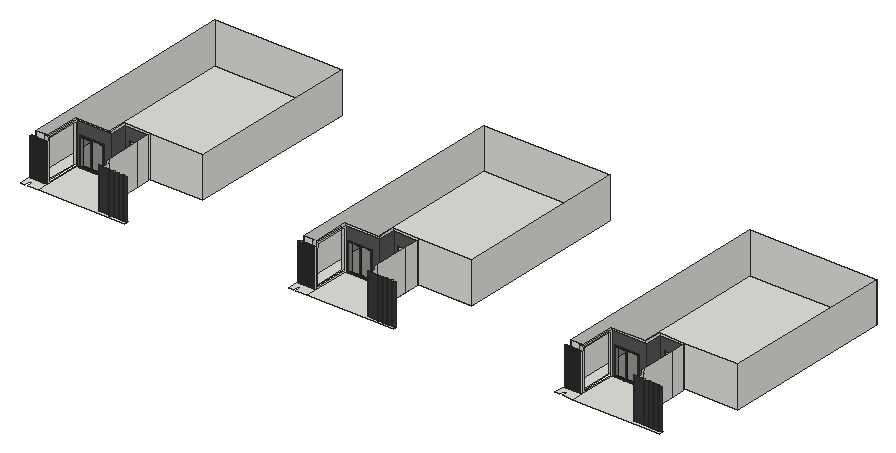
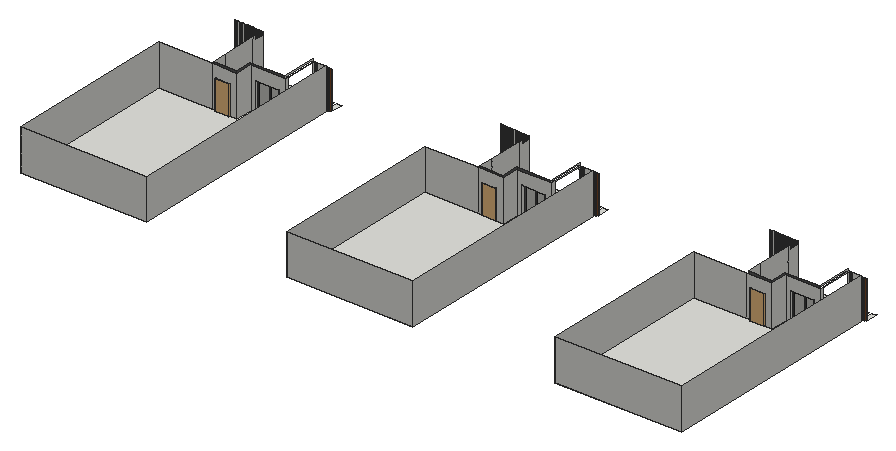
# SketchUp Ruby script. Lengths in inches.
U = 1.inch
M = Sketchup.active_model
def pt(a) = Geom::Point3d.new(a.map { |v| v * U })
def face(e, loops, mat)
  f = e.add_face(loops[0].map { |a| pt(a) })
  loops[1..].each { |l| e.add_face(l.map { |a| pt(a) }).erase! }
  f.material = f.back_material = mat if mat
  f
end
# faces: each face lists its corners as indices into pts; further lists are holes
def faces(e, pts, list, mat = nil) = list.each { |f| face(e, (f[0].is_a?(Array) ? f : [f]).map { |l| l.map { |i| pts[i] } }, mat) }
# xy, xz, yz: faces in a plane at the given z, y or x. An outline is a flat list of corners, or four numbers for a rectangle; further outlines are holes
def ring(l) = l.size == 4 ? [[l[0], l[1]], [l[2], l[1]], [l[2], l[3]], [l[0], l[3]]] : l.each_slice(2).to_a
def flat(e, list, mat, &to3) = list.each { |f| face(e, (f[0].is_a?(Array) ? f : [f]).map { |l| ring(l).map { |u, v| to3.(u, v) } }, mat) }
def xy(e, z, list, mat = nil) = flat(e, list, mat) { |x, y| [x, y, z] }
def xz(e, y, list, mat = nil) = flat(e, list, mat) { |x, z| [x, y, z] }
def yz(e, x, list, mat = nil) = flat(e, list, mat) { |y, z| [x, y, z] }
def lines(e, pts, list) = list.each { |a, b| e.add_line(pt(pts[a]), pt(pts[b])) }
# prism: a flat outline (further loops are holes) pulled along v
def prism(e, loops, v, mat = nil)
  f = face(e, loops, mat); d = Geom::Vector3d.new(v.map { |x| x * U })
  f.pushpull(f.normal.samedirection?(d) ? d.length : -d.length)
end
def box(e, o, s, mat = nil) = prism(e, [[o, [o[0] + s[0], o[1], o[2]], [o[0] + s[0], o[1] + s[1], o[2]], [o[0], o[1] + s[1], o[2]]]], [0, 0, s[2]], mat)
def at(x, y, z, deg = 0) = Geom::Transformation.translation(pt([x, y, z])) * Geom::Transformation.rotation(ORIGIN, Z_AXIS, deg.degrees)
def axes(o, x, y, z) = Geom::Transformation.new([*x, 0, *y, 0, *z, 0, *pt(o).to_a, 1])
def part(name) = M.definitions.add(name)
# library, detail: a bought-in or finely detailed component or shape, given as its bounding box
def library(name, o, s) = part(name).tap { |d| box(d.entities, o, s) }
def detail(e, o, s) = box(e.add_group.entities, o, s)
def put(e, d, t, mat = nil) = e.add_instance(d, t).tap { |i| i.material = mat if mat }
def group(e, t, mat = nil) = e.add_group.tap { |g| g.transformation = t; g.material = mat if mat }.entities
root = M.entities
M.materials.add("Glass_Tinted_Gray").color = [0, 0, 0]
M.materials["Glass_Tinted_Gray"].alpha = 0.125
M.materials.add("[0135_DarkGray]").color = [81, 81, 81]
M.materials.add("[Color M06]").color = [86, 86, 86]
M.materials.add("[Color M07]").color = [58, 58, 58]
M.materials.add("[Mirror 02]").color = [229, 229, 229]
M.materials.add("[Terrazzo Light Blue]").color = [196, 214, 227]
M.materials.add("[Wood Veneer 01]").color = [120, 70, 37]
c1 = part("PENTEK_RP Fineline 50S_Sliding_DoorCase_E1")
box(c1.entities,[0,0,0],[1.51,3.66,99.27],"[0135_DarkGray]")
c2 = part("PENTEK_RP Fineline 50S_SlidingDooe_Case_E2")
box(c2.entities,[0,0,0],[96.25,3.66,1.51],"[0135_DarkGray]")
c3 = part("pentek_RP Fineline 50S_SlidingDoor_Case")
put(c3.entities,c1,at(97.76,0,0))
put(c3.entities,c2,at(1.51,0,0))
put(c3.entities,c1,at(0,0,0))
put(c3.entities,c2,at(1.51,0,97.76))
c4 = part("PENTEK_RP Fineline 50S_SlidingDoor_GlazingBead_2")
box(c4.entities,[0,0,0],[0.56,0.59,94.39],"[0135_DarkGray]")
c5 = part("PENTEK_RP Fineline 50S_SlidingDoor_Glass")
box(c5.entities,[0,0,0],[46.58,0.16,94.39],"Glass_Tinted_Gray")
c6 = part("PENTEK_RP Fineline 50S_SlidingDoor_GlazingBead")
box(c6.entities,[0,0,0],[45.47,0.59,0.56],"[0135_DarkGray]")
c7 = part("PENTEK_RP Fineline 50S_SlidingDoor_Leaf_E1")
xy(c7.entities,0,[[0,0,0.93,1.97],[0.93,1.57,1.49,1.97]],"[0135_DarkGray]")
xy(c7.entities,96.25,[[0,0,0.93,0,0.93,1.57,1.49,1.57,1.49,1.97,0,1.97]],"[0135_DarkGray]")
xz(c7.entities,0,[[0,0,0.93,96.25]],"[0135_DarkGray]")
xz(c7.entities,1.57,[[0.93,0,1.49,95.32],[0.93,95.32,1.49,96.25]],"[0135_DarkGray]")
xz(c7.entities,1.97,[[0,0,1.49,96.25]],"[0135_DarkGray]")
yz(c7.entities,0,[[0,0,1.97,96.25]],"[0135_DarkGray]")
yz(c7.entities,0.93,[[0,0,1.57,0.93],[0,0.93,1.57,95.32],[0,95.32,1.57,96.25]],"[0135_DarkGray]")
yz(c7.entities,1.49,[[1.57,0,1.97,95.32],[1.57,95.32,1.97,96.25]],"[0135_DarkGray]")
c8 = part("PENTEK_RP Fineline 50S_SlidingDoor_Leaf_E2")
xy(c8.entities,0,[[0,0,0,1.57,0.56,1.57,0.56,1.97,46.02,1.97,46.02,1.57,46.58,1.57,46.58,0]],"[0135_DarkGray]")
xy(c8.entities,0.93,[[0,0,46.58,1.57]],"[0135_DarkGray]")
xy(c8.entities,1.49,[[0.56,1.57,46.02,1.97]],"[0135_DarkGray]")
xz(c8.entities,0,[[0,0,46.58,0.93]],"[0135_DarkGray]")
xz(c8.entities,1.57,[[0,0,0.56,0.93],[46.02,0,46.58,0.93],[0.56,0.93,46.02,1.49]],"[0135_DarkGray]")
xz(c8.entities,1.97,[[0.56,0,46.02,1.49]],"[0135_DarkGray]")
yz(c8.entities,0,[[0,0,1.57,0.93]],"[0135_DarkGray]")
yz(c8.entities,0.56,[[1.57,0,1.97,0.93],[1.57,0.93,1.97,1.49]],"[0135_DarkGray]")
yz(c8.entities,46.02,[[1.57,0,1.97,0.93],[1.57,0.93,1.97,1.49]],"[0135_DarkGray]")
yz(c8.entities,46.58,[[0,0,1.57,0.93]],"[0135_DarkGray]")
c9 = part("PENTEK_RP Fineline S_SlidingDoor_Leaf1")
put(c9.entities,c4,at(0.93,0,0.93))
put(c9.entities,c4,at(46.96,0,0.93))
put(c9.entities,c5,at(1.49,1.42,0.93))
put(c9.entities,c6,at(1.49,0,0.93))
put(c9.entities,c5,at(1.49,0.59,0.93),"[Terrazzo Light Blue]")
put(c9.entities,c7,at(0,0,0))
put(c9.entities,c7,axes([48.44,0,0],[-1,0,0],[0,1,0],[0,0,1]))
put(c9.entities,c8,axes([0.93,0,96.25],[1,0,0],[0,1,0],[0,0,-1]))
put(c9.entities,c8,at(0.93,0,0))
put(c9.entities,c6,at(1.49,0,94.77))
c10 = part("PENTEK_RP Fineline 50S_SlidingDoor_Leaf2")
put(c10.entities,c5,at(1.49,1.42,0.93))
put(c10.entities,c6,at(1.49,0,94.77))
put(c10.entities,c4,at(46.96,0,0.93))
put(c10.entities,c5,at(1.49,0.59,0.93),"[Mirror 02]")
put(c10.entities,c4,at(0.93,0,0.93))
put(c10.entities,c7,at(0,0,0))
put(c10.entities,c7,axes([48.44,0,0],[-1,0,0],[0,1,0],[0,0,1]))
put(c10.entities,c6,at(1.49,0,0.93))
put(c10.entities,c8,axes([0.93,0,96.25],[1,0,0],[0,1,0],[0,0,-1]))
put(c10.entities,c8,at(0.93,0,0))
c11 = part("PENTEK - Slimmest Steel Sliding Door / Window\#1")
put(c11.entities,c3,at(0,-1.88,-0.09))
put(c11.entities,c9,at(1.51,-2.27,1.42))
put(c11.entities,c10,at(49.32,-0.3,1.42))
c12 = library("door (1)",[38.93,25.48,0],[40,9.94,82.68])
xy(root,273.625,[[874.71,264.125,888.27,264.125,888.27,279.8125,895.625,279.8125,895.625,264.125,927.52,264.125,927.52,300.5625,924.42,300.5625,924.42,297.375,920.81,297.375,920.81,300.5625,919.9375,300.5625,919.9375,297.375,916.32,297.375,916.32,300.5625,915.46,300.5625,915.46,297.375,911.84,297.375,911.84,300.5625,910.89,300.5625,910.89,297.375,907.28,297.375,907.28,300.5625,905.86,300.5625,905.86,297.375,902.25,297.375,902.25,300.5625,900.83,300.5625,900.83,297.375,897.21,297.375,897.21,301,896.33,301,896.33,297.375,892.71,297.375,892.71,301,891.83,301,891.83,297.375,888.21,297.375,888.21,301,887.33,301,887.33,297.375,883.71,297.375,883.71,301,882.83,301,882.83,297.375,879.21,297.375,879.21,301,878.33,301,878.33,297.375,874.71,297.375],[927.52,264.125,1181.97,264.125,1181.97,271.6875,1171.33,271.6875,1171.33,273.0625,1169.74,273.0625,1169.74,271.6875,1157.32,271.6875,1157.32,273.0625,1155.73,273.0625,1155.73,271.6875,1143.3,271.6875,1143.3,273.0625,1141.72,273.0625,1141.72,271.6875,1129.29,271.6875,1129.29,273.0625,1098.03,273.0625,1098.03,452.5625,1084.66,452.97,1084.91,461.29,1043.56,462.56,1043.3,454.25,1029.02,454.6875,1029.02,405,1006.52,405,1006.52,413.31,938.52,413.31,938.52,405,927.52,405],[1661.09,264.125,1674.65,264.125,1674.65,279.8125,1682,279.8125,1682,264.125,1713.9,264.125,1713.9,300.5625,1710.79,300.5625,1710.79,297.375,1707.18,297.375,1707.18,300.5625,1706.3125,300.5625,1706.3125,297.375,1702.7,297.375,1702.7,300.5625,1701.83,300.5625,1701.83,297.375,1698.22,297.375,1698.22,300.5625,1697.27,300.5625,1697.27,297.375,1693.66,297.375,1693.66,300.5625,1692.23,300.5625,1692.23,297.375,1688.62,297.375,1688.62,300.5625,1687.2,300.5625,1687.2,297.375,1683.59,297.375,1683.59,301,1682.7,301,1682.7,297.375,1679.09,297.375,1679.09,301,1678.2,301,1678.2,297.375,1674.59,297.375,1674.59,301,1673.7,301,1673.7,297.375,1670.09,297.375,1670.09,301,1669.2,301,1669.2,297.375,1665.59,297.375,1665.59,301,1664.7,301,1664.7,297.375,1661.09,297.375],[1713.9,264.125,1968.34,264.125,1968.34,271.6875,1957.7,271.6875,1957.7,273.0625,1956.12,273.0625,1956.12,271.6875,1943.69,271.6875,1943.69,273.0625,1942.11,273.0625,1942.11,271.6875,1929.68,271.6875,1929.68,273.0625,1928.09,273.0625,1928.09,271.6875,1915.67,271.6875,1915.67,273.0625,1884.4,273.0625,1884.4,452.5625,1871.03,452.97,1871.29,461.29,1829.93,462.56,1829.68,454.25,1815.4,454.6875,1815.4,405,1792.89,405,1792.89,413.31,1724.89,413.31,1724.89,405,1713.9,405],[2441.46,264.125,2455.02,264.125,2455.02,279.8125,2462.375,279.8125,2462.375,264.125,2494.27,264.125,2494.27,300.5625,2491.17,300.5625,2491.17,297.375,2487.56,297.375,2487.56,300.5625,2486.6875,300.5625,2486.6875,297.375,2483.07,297.375,2483.07,300.5625,2482.21,300.5625,2482.21,297.375,2478.59,297.375,2478.59,300.5625,2477.64,300.5625,2477.64,297.375,2474.03,297.375,2474.03,300.5625,2472.61,300.5625,2472.61,297.375,2469,297.375,2469,300.5625,2467.58,300.5625,2467.58,297.375,2463.96,297.375,2463.96,301,2463.08,301,2463.08,297.375,2459.46,297.375,2459.46,301,2458.58,301,2458.58,297.375,2454.96,297.375,2454.96,301,2454.08,301,2454.08,297.375,2450.46,297.375,2450.46,301,2449.58,301,2449.58,297.375,2445.96,297.375,2445.96,301,2445.08,301,2445.08,297.375,2441.46,297.375],
  [2494.27,264.125,2748.72,264.125,2748.72,271.6875,2738.08,271.6875,2738.08,273.0625,2736.49,273.0625,2736.49,271.6875,2724.07,271.6875,2724.07,273.0625,2722.48,273.0625,2722.48,271.6875,2710.05,271.6875,2710.05,273.0625,2708.47,273.0625,2708.47,271.6875,2696.04,271.6875,2696.04,273.0625,2664.78,273.0625,2664.78,452.5625,2651.41,452.97,2651.66,461.29,2610.31,462.56,2610.05,454.25,2595.77,454.6875,2595.77,405,2573.27,405,2573.27,413.31,2505.27,413.31,2505.27,405,2494.27,405],[1129.29,271.6875,1141.72,273.0625],[1143.3,271.6875,1155.73,273.0625],[1157.32,271.6875,1169.74,273.0625],[1171.33,271.6875,1181.97,273.0625],
  [1915.67,271.6875,1928.09,273.0625],[1929.68,271.6875,1942.11,273.0625],[1943.69,271.6875,1956.12,273.0625],[1957.7,271.6875,1968.34,273.0625],[2696.04,271.6875,2708.47,273.0625],
  [2710.05,271.6875,2722.48,273.0625],[2724.07,271.6875,2736.49,273.0625],[2738.08,271.6875,2748.72,273.0625],[902.25,297.375,905.86,301],[1688.62,297.375,1692.23,301],
  [2469,297.375,2472.61,301],[883.03,309.31,919.21,309.31,919.21,413.31,1020.71,413.31,1020.71,463.26,1043.56,462.56,1084.91,461.29,1098.16,460.88,1252.27,460.88,1252.27,967.62,883.03,967.62],[1669.4,309.31,1705.58,309.31,1705.58,413.31,1807.08,413.31,1807.08,463.26,1829.93,462.56,1871.29,461.29,1884.53,460.88,2038.65,460.88,2038.65,967.62,1669.4,967.62],[2449.78,309.31,2485.96,309.31,2485.96,413.31,2587.46,413.31,2587.46,463.26,2610.31,462.56,2651.66,461.29,2664.91,460.88,2819.02,460.88,2819.02,967.62,2449.78,967.62]])
xz(root,271.6875,[[1129.29,273.625,1141.72,393.625],[1143.3,273.625,1155.73,393.625],[1157.32,273.625,1169.74,393.625],[1171.33,273.625,1181.97,393.625],[1915.67,273.625,1928.09,393.625],
  [1929.68,273.625,1942.11,393.625],[1943.69,273.625,1956.12,393.625],[1957.7,273.625,1968.34,393.625],[2696.04,273.625,2708.47,393.625],[2710.05,273.625,2722.48,393.625],
  [2724.07,273.625,2736.49,393.625],[2738.08,273.625,2748.72,393.625]],"[Color M07]")
xz(root,273.0625,[[1098.03,273.625,1129.29,393.625],[1141.72,273.625,1143.3,393.625],[1155.73,273.625,1157.32,393.625],[1169.74,273.625,1171.33,393.625],[1884.4,273.625,1915.67,393.625],
  [1928.09,273.625,1929.68,393.625],[1942.11,273.625,1943.69,393.625],[1956.12,273.625,1957.7,393.625],[2664.78,273.625,2696.04,393.625],[2708.47,273.625,2710.05,393.625],
  [2722.48,273.625,2724.07,393.625],[2736.49,273.625,2738.08,393.625]],"[Color M07]")
xz(root,297.375,[[874.71,273.625,878.33,382.6875],[879.21,273.625,882.83,382.6875],[883.71,273.625,887.33,382.6875],[888.21,273.625,891.83,382.6875],[892.71,273.625,896.33,382.6875],
  [897.21,273.625,900.83,382.6875],[902.25,273.625,905.86,382.28],[907.28,273.625,910.89,382.28],[911.84,273.625,915.46,382.28],[916.32,273.625,919.9375,382.28],
  [920.81,273.625,924.42,382.28],[1661.09,273.625,1664.7,382.6875],[1665.59,273.625,1669.2,382.6875],[1670.09,273.625,1673.7,382.6875],[1674.59,273.625,1678.2,382.6875],
  [1679.09,273.625,1682.7,382.6875],[1683.59,273.625,1687.2,382.6875],[1688.62,273.625,1692.23,382.28],[1693.66,273.625,1697.27,382.28],[1698.22,273.625,1701.83,382.28],
  [1702.7,273.625,1706.3125,382.28],[1707.18,273.625,1710.79,382.28],[2441.46,273.625,2445.08,382.6875],[2445.96,273.625,2449.58,382.6875],[2450.46,273.625,2454.08,382.6875],
  [2454.96,273.625,2458.58,382.6875],[2459.46,273.625,2463.08,382.6875],[2463.96,273.625,2467.58,382.6875],[2469,273.625,2472.61,382.28],[2474.03,273.625,2477.64,382.28],
  [2478.59,273.625,2482.21,382.28],[2483.07,273.625,2486.6875,382.28],[2487.56,273.625,2491.17,382.28]],"[Wood Veneer 01]")
xz(root,300.5625,[[900.83,273.625,902.25,273.625,902.25,382.28,905.86,382.28,905.86,273.625,907.28,273.625,907.28,382.28,910.89,382.28,910.89,273.625,911.84,273.625,911.84,382.28,915.46,382.28,915.46,273.625,916.32,273.625,916.32,382.28,919.9375,382.28,919.9375,273.625,920.81,273.625,920.81,382.28,924.42,382.28,924.42,273.625,927.52,273.625,927.52,382.6875,900.83,382.6875],[1687.2,273.625,1688.62,273.625,1688.62,382.28,1692.23,382.28,1692.23,273.625,1693.66,273.625,1693.66,382.28,1697.27,382.28,1697.27,273.625,1698.22,273.625,1698.22,382.28,1701.83,382.28,1701.83,273.625,1702.7,273.625,1702.7,382.28,1706.3125,382.28,1706.3125,273.625,1707.18,273.625,1707.18,382.28,1710.79,382.28,1710.79,273.625,1713.9,273.625,1713.9,382.6875,1687.2,382.6875],[2467.58,273.625,2469,273.625,2469,382.28,2472.61,382.28,2472.61,273.625,2474.03,273.625,2474.03,382.28,2477.64,382.28,2477.64,273.625,2478.59,273.625,2478.59,382.28,2482.21,382.28,2482.21,273.625,2483.07,273.625,2483.07,382.28,2486.6875,382.28,2486.6875,273.625,2487.56,273.625,2487.56,382.28,2491.17,382.28,2491.17,273.625,2494.27,273.625,2494.27,382.6875,2467.58,382.6875]],"[Wood Veneer 01]")
xz(root,301,[[902.25,273.22,905.86,273.625],[1688.62,273.22,1692.23,273.625],[2469,273.22,2472.61,273.625],[878.33,273.625,879.21,382.6875],[1664.7,273.625,1665.59,382.6875],
  [2445.08,273.625,2445.96,382.6875]])
xz(root,301,[[882.83,273.625,883.71,382.6875],[887.33,273.625,888.21,382.6875],[891.83,273.625,892.71,382.6875],[896.33,273.625,897.21,382.6875],[1669.2,273.625,1670.09,382.6875],
  [1673.7,273.625,1674.59,382.6875],[1678.2,273.625,1679.09,382.6875],[1682.7,273.625,1683.59,382.6875],[2449.58,273.625,2450.46,382.6875],[2454.08,273.625,2454.96,382.6875],
  [2458.58,273.625,2459.46,382.6875],[2463.08,273.625,2463.96,382.6875]],"[Wood Veneer 01]")
xz(root,309.31,[[883.03,273.625,883.03,393.625,919.21,393.625,919.21,391.8,907.08,391.8,907.08,275.45,919.21,275.45,919.21,273.625],[1669.4,273.625,1669.4,393.625,1705.58,393.625,1705.58,391.8,1693.46,391.8,1693.46,275.45,1705.58,275.45,1705.58,273.625],[2449.78,273.625,2449.78,393.625,2485.96,393.625,2485.96,391.8,2473.83,391.8,2473.83,275.45,2485.96,275.45,2485.96,273.625]])
xz(root,405,[[927.52,273.625,938.52,273.625,938.52,357.625,1006.52,357.625,1006.52,273.625,1029.02,273.625,1029.02,393.625,927.52,393.625],[1713.9,273.625,1724.89,273.625,1724.89,357.625,1792.89,357.625,1792.89,273.625,1815.4,273.625,1815.4,393.625,1713.9,393.625],[2494.27,273.625,2505.27,273.625,2505.27,357.625,2573.27,357.625,2573.27,273.625,2595.77,273.625,2595.77,393.625,2494.27,393.625]],"[Color M06]")
xz(root,413.31,[[919.21,273.625,919.21,393.625,1020.71,393.625,1020.71,273.625,1006.52,273.625,1006.52,357.625,938.52,357.625,938.52,273.625],[1705.58,273.625,1705.58,393.625,1807.08,393.625,1807.08,273.625,1792.89,273.625,1792.89,357.625,1724.89,357.625,1724.89,273.625],[2485.96,273.625,2485.96,393.625,2587.46,393.625,2587.46,273.625,2573.27,273.625,2573.27,357.625,2505.27,357.625,2505.27,273.625]])
xz(root,460.88,[[1098.16,273.625,1252.27,393.625],[1884.53,273.625,2038.65,393.625],[2664.91,273.625,2819.02,393.625]])
xz(root,967.62,[[883.03,273.625,1252.27,393.625],[1669.4,273.625,2038.65,393.625],[2449.78,273.625,2819.02,393.625]])
yz(root,878.33,[[297.375,273.625,301,382.6875]],"[Wood Veneer 01]")
yz(root,879.21,[[297.375,273.625,301,382.6875]])
yz(root,882.83,[[297.375,273.625,301,382.6875]],"[Wood Veneer 01]")
yz(root,883.03,[[309.31,273.625,967.62,393.625]])
yz(root,883.71,[[297.375,273.625,301,382.6875]])
yz(root,887.33,[[297.375,273.625,301,382.6875]])
yz(root,888.21,[[297.375,273.625,301,382.6875]])
yz(root,891.83,[[297.375,273.625,301,382.6875]])
yz(root,892.71,[[297.375,273.625,301,382.6875]])
yz(root,896.33,[[297.375,273.625,301,382.6875]])
yz(root,897.21,[[297.375,273.625,301,382.6875]])
yz(root,900.83,[[297.375,273.625,300.5625,382.6875]])
yz(root,902.25,[[297.375,273.625,300.5625,382.28]])
yz(root,905.86,[[297.375,273.625,300.5625,382.28]])
yz(root,907.28,[[297.375,273.625,300.5625,382.28]])
yz(root,910.89,[[297.375,273.625,300.5625,382.28]])
yz(root,911.84,[[297.375,273.625,300.5625,382.28]])
yz(root,915.46,[[297.375,273.625,300.5625,382.28]])
yz(root,916.32,[[297.375,273.625,300.5625,382.28]])
yz(root,919.21,[[309.31,273.625,309.31,275.45,403.18,275.45,403.18,391.8,309.31,391.8,309.31,393.625,413.31,393.625,413.31,273.625]])
yz(root,919.9375,[[297.375,273.625,300.5625,382.28]])
yz(root,920.81,[[297.375,273.625,300.5625,382.28]])
yz(root,924.42,[[297.375,273.625,300.5625,382.28]])
yz(root,927.52,[[[300.5625,273.625,405,273.625,405,393.625,301,393.625,301,382.6875,300.5625,382.6875],[302.38,275.45,302.38,380.87,302.82,380.87,302.82,391.8,403.18,391.8,403.18,275.45]]])
yz(root,938.52,[[405,273.625,413.31,357.625]])
yz(root,1006.52,[[405,273.625,413.31,357.625]])
yz(root,1020.71,[[413.31,273.625,463.26,393.625]])
yz(root,1029.02,[[405,273.625,454.6875,393.625]],"[Color M06]")
yz(root,1098.03,[[273.0625,273.625,273.0625,382.6875,301,382.6875,301,393.625,308.24,393.625,308.24,273.625],[308.24,273.625,411.0625,393.625],[411.0625,273.625,452.5625,393.625]])
yz(root,1129.29,[[271.6875,273.625,273.0625,393.625]])
yz(root,1141.72,[[271.6875,273.625,273.0625,393.625]])
yz(root,1143.3,[[271.6875,273.625,273.0625,393.625]])
yz(root,1155.73,[[271.6875,273.625,273.0625,393.625]])
yz(root,1157.32,[[271.6875,273.625,273.0625,393.625]])
yz(root,1169.74,[[271.6875,273.625,273.0625,393.625]])
yz(root,1171.33,[[271.6875,273.625,273.0625,393.625]])
yz(root,1252.27,[[460.88,273.625,967.62,393.625]])
yz(root,1664.7,[[297.375,273.625,301,382.6875]],"[Wood Veneer 01]")
yz(root,1665.59,[[297.375,273.625,301,382.6875]])
yz(root,1669.2,[[297.375,273.625,301,382.6875]],"[Wood Veneer 01]")
yz(root,1669.4,[[309.31,273.625,967.62,393.625]])
yz(root,1670.09,[[297.375,273.625,301,382.6875]])
yz(root,1673.7,[[297.375,273.625,301,382.6875]])
yz(root,1674.59,[[297.375,273.625,301,382.6875]])
yz(root,1678.2,[[297.375,273.625,301,382.6875]])
yz(root,1679.09,[[297.375,273.625,301,382.6875]])
yz(root,1682.7,[[297.375,273.625,301,382.6875]])
yz(root,1683.59,[[297.375,273.625,301,382.6875]])
yz(root,1687.2,[[297.375,273.625,300.5625,382.6875]])
yz(root,1688.62,[[297.375,273.625,300.5625,382.28]])
yz(root,1692.23,[[297.375,273.625,300.5625,382.28]])
yz(root,1693.66,[[297.375,273.625,300.5625,382.28]])
yz(root,1697.27,[[297.375,273.625,300.5625,382.28]])
yz(root,1698.22,[[297.375,273.625,300.5625,382.28]])
yz(root,1701.83,[[297.375,273.625,300.5625,382.28]])
yz(root,1702.7,[[297.375,273.625,300.5625,382.28]])
yz(root,1705.58,[[309.31,273.625,309.31,275.45,403.18,275.45,403.18,391.8,309.31,391.8,309.31,393.625,413.31,393.625,413.31,273.625]])
yz(root,1706.3125,[[297.375,273.625,300.5625,382.28]])
yz(root,1707.18,[[297.375,273.625,300.5625,382.28]])
yz(root,1710.79,[[297.375,273.625,300.5625,382.28]])
yz(root,1713.9,[[[300.5625,273.625,405,273.625,405,393.625,301,393.625,301,382.6875,300.5625,382.6875],[302.38,275.45,302.38,380.87,302.82,380.87,302.82,391.8,403.18,391.8,403.18,275.45]]])
yz(root,1724.89,[[405,273.625,413.31,357.625]])
yz(root,1792.89,[[405,273.625,413.31,357.625]])
yz(root,1807.08,[[413.31,273.625,463.26,393.625]])
yz(root,1815.4,[[405,273.625,454.6875,393.625]],"[Color M06]")
yz(root,1884.4,[[273.0625,273.625,273.0625,382.6875,301,382.6875,301,393.625,308.24,393.625,308.24,273.625],[308.24,273.625,411.0625,393.625],[411.0625,273.625,452.5625,393.625]])
yz(root,1915.67,[[271.6875,273.625,273.0625,393.625]])
yz(root,1928.09,[[271.6875,273.625,273.0625,393.625]])
yz(root,1929.68,[[271.6875,273.625,273.0625,393.625]])
yz(root,1942.11,[[271.6875,273.625,273.0625,393.625]])
yz(root,1943.69,[[271.6875,273.625,273.0625,393.625]])
yz(root,1956.12,[[271.6875,273.625,273.0625,393.625]])
yz(root,1957.7,[[271.6875,273.625,273.0625,393.625]])
yz(root,2038.65,[[460.88,273.625,967.62,393.625]])
yz(root,2445.08,[[297.375,273.625,301,382.6875]],"[Wood Veneer 01]")
yz(root,2445.96,[[297.375,273.625,301,382.6875]])
yz(root,2449.58,[[297.375,273.625,301,382.6875]],"[Wood Veneer 01]")
yz(root,2449.78,[[309.31,273.625,967.62,393.625]])
yz(root,2450.46,[[297.375,273.625,301,382.6875]])
yz(root,2454.08,[[297.375,273.625,301,382.6875]])
yz(root,2454.96,[[297.375,273.625,301,382.6875]])
yz(root,2458.58,[[297.375,273.625,301,382.6875]])
yz(root,2459.46,[[297.375,273.625,301,382.6875]])
yz(root,2463.08,[[297.375,273.625,301,382.6875]])
yz(root,2463.96,[[297.375,273.625,301,382.6875]])
yz(root,2467.58,[[297.375,273.625,300.5625,382.6875]])
yz(root,2469,[[297.375,273.625,300.5625,382.28]])
yz(root,2472.61,[[297.375,273.625,300.5625,382.28]])
yz(root,2474.03,[[297.375,273.625,300.5625,382.28]])
yz(root,2477.64,[[297.375,273.625,300.5625,382.28]])
yz(root,2478.59,[[297.375,273.625,300.5625,382.28]])
yz(root,2482.21,[[297.375,273.625,300.5625,382.28]])
yz(root,2483.07,[[297.375,273.625,300.5625,382.28]])
yz(root,2485.96,[[309.31,273.625,309.31,275.45,403.18,275.45,403.18,391.8,309.31,391.8,309.31,393.625,413.31,393.625,413.31,273.625]])
yz(root,2486.6875,[[297.375,273.625,300.5625,382.28]])
yz(root,2487.56,[[297.375,273.625,300.5625,382.28]])
yz(root,2491.17,[[297.375,273.625,300.5625,382.28]])
yz(root,2494.27,[[[300.5625,273.625,405,273.625,405,393.625,301,393.625,301,382.6875,300.5625,382.6875],[302.38,275.45,302.38,380.87,302.82,380.87,302.82,391.8,403.18,391.8,403.18,275.45]]])
yz(root,2505.27,[[405,273.625,413.31,357.625]])
yz(root,2573.27,[[405,273.625,413.31,357.625]])
yz(root,2587.46,[[413.31,273.625,463.26,393.625]])
yz(root,2595.77,[[405,273.625,454.6875,393.625]],"[Color M06]")
yz(root,2664.78,[[273.0625,273.625,273.0625,382.6875,301,382.6875,301,393.625,308.24,393.625,308.24,273.625],[308.24,273.625,411.0625,393.625],[411.0625,273.625,452.5625,393.625]])
yz(root,2696.04,[[271.6875,273.625,273.0625,393.625]])
yz(root,2708.47,[[271.6875,273.625,273.0625,393.625]])
yz(root,2710.05,[[271.6875,273.625,273.0625,393.625]])
yz(root,2722.48,[[271.6875,273.625,273.0625,393.625]])
yz(root,2724.07,[[271.6875,273.625,273.0625,393.625]])
yz(root,2736.49,[[271.6875,273.625,273.0625,393.625]])
yz(root,2738.08,[[271.6875,273.625,273.0625,393.625]])
yz(root,2819.02,[[460.88,273.625,967.62,393.625]])
p = [[1029.02,454.6875,273.625],[1043.3,454.25,273.625],[1043.3,454.25,358.5],[1084.66,452.97,358.5],[1084.66,452.97,273.625],[1098.03,452.5625,273.625],
  [1098.03,452.5625,393.625],[1029.02,454.6875,393.625],[1815.4,454.6875,273.625],[1829.68,454.25,273.625],[1829.68,454.25,358.5],[1871.03,452.97,358.5],
  [1871.03,452.97,273.625],[1884.4,452.5625,273.625],[1884.4,452.5625,393.625],[1815.4,454.6875,393.625],[2595.77,454.6875,273.625],[2610.05,454.25,273.625],
  [2610.05,454.25,358.5],[2651.41,452.97,358.5],[2651.41,452.97,273.625],[2664.78,452.5625,273.625],[2664.78,452.5625,393.625],[2595.77,454.6875,393.625],
  [1084.91,461.29,358.5],[1084.91,461.29,273.625],[1871.29,461.29,358.5],[1871.29,461.29,273.625],[2651.66,461.29,358.5],[2651.66,461.29,273.625],
  [1043.56,462.56,273.625],[1043.56,462.56,358.5],[1829.93,462.56,273.625],[1829.93,462.56,358.5],[2610.31,462.56,273.625],[2610.31,462.56,358.5],
  [1020.71,463.26,273.625],[1020.71,463.26,393.625],[1098.16,460.88,393.625],[1098.16,460.88,273.625],[1807.08,463.26,273.625],[1807.08,463.26,393.625],
  [1884.53,460.88,393.625],[1884.53,460.88,273.625],[2587.46,463.26,273.625],[2587.46,463.26,393.625],[2664.91,460.88,393.625],[2664.91,460.88,273.625]]
faces(root,p,[[0,1,2,3,4,5,6,7],[8,9,10,11,12,13,14,15],[16,17,18,19,20,21,22,23]],"[Color M06]")
faces(root,p,[[4,3,24,25],[12,11,26,27],[20,19,28,29],[2,1,30,31],[10,9,32,33],[18,17,34,35],[30,36,37,38,39,25,24,31],[32,40,41,42,43,27,26,33],
  [34,44,45,46,47,29,28,35]])
put(root,c11,axes([1722.64,405.56,273.61],[0.6868,0,0],[0,0.6868,0],[0,0,0.85163]))
put(root,c11,axes([936.27,405.56,273.61],[0.6868,0,0],[0,0.6868,0],[0,0,0.85163]))
put(root,c11,axes([2503.02,405.56,273.61],[0.6868,0,0],[0,0.6868,0],[0,0,0.85163]))
put(root,c12,axes([1789.43,428.76,273.625],[1.03388,0,0],[0,1,0],[0,0,1.02658]))
put(root,c12,axes([1003.06,428.76,273.625],[1.03388,0,0],[0,1,0],[0,0,1.02658]))
put(root,c12,axes([2569.81,428.76,273.625],[1.03388,0,0],[0,1,0],[0,0,1.02658]))
